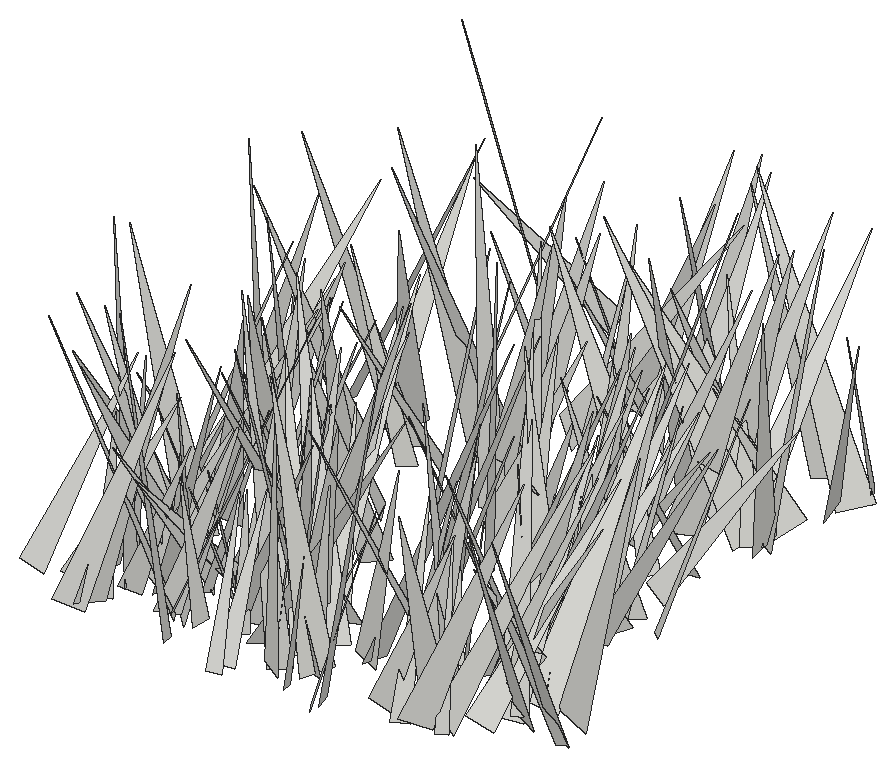
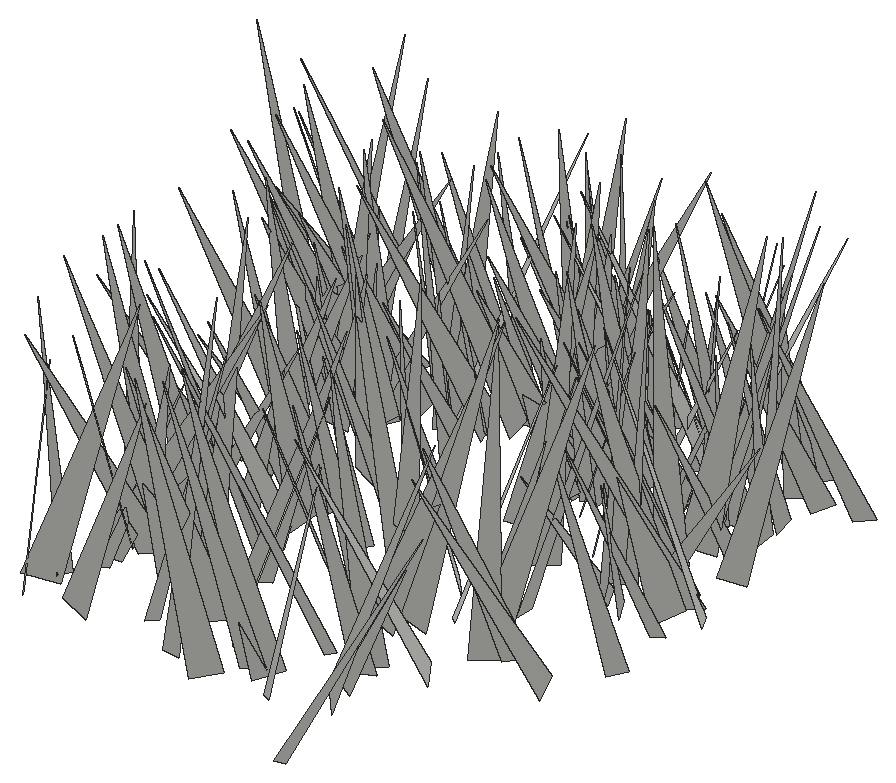
# SketchUp Ruby script. Lengths in inches.
U = 1.inch
M = Sketchup.active_model
def pt(a) = Geom::Point3d.new(a.map { |v| v * U })
def face(e, loops, mat)
  f = e.add_face(loops[0].map { |a| pt(a) })
  loops[1..].each { |l| e.add_face(l.map { |a| pt(a) }).erase! }
  f.material = f.back_material = mat if mat
  f
end
# faces: each face lists its corners as indices into pts; further lists are holes
def faces(e, pts, list, mat = nil) = list.each { |f| face(e, (f[0].is_a?(Array) ? f : [f]).map { |l| l.map { |i| pts[i] } }, mat) }
# xy, xz, yz: faces in a plane at the given z, y or x. An outline is a flat list of corners, or four numbers for a rectangle; further outlines are holes
def ring(l) = l.size == 4 ? [[l[0], l[1]], [l[2], l[1]], [l[2], l[3]], [l[0], l[3]]] : l.each_slice(2).to_a
def flat(e, list, mat, &to3) = list.each { |f| face(e, (f[0].is_a?(Array) ? f : [f]).map { |l| ring(l).map { |u, v| to3.(u, v) } }, mat) }
def xy(e, z, list, mat = nil) = flat(e, list, mat) { |x, y| [x, y, z] }
def xz(e, y, list, mat = nil) = flat(e, list, mat) { |x, z| [x, y, z] }
def yz(e, x, list, mat = nil) = flat(e, list, mat) { |y, z| [x, y, z] }
def lines(e, pts, list) = list.each { |a, b| e.add_line(pt(pts[a]), pt(pts[b])) }
# prism: a flat outline (further loops are holes) pulled along v
def prism(e, loops, v, mat = nil)
  f = face(e, loops, mat); d = Geom::Vector3d.new(v.map { |x| x * U })
  f.pushpull(f.normal.samedirection?(d) ? d.length : -d.length)
end
def box(e, o, s, mat = nil) = prism(e, [[o, [o[0] + s[0], o[1], o[2]], [o[0] + s[0], o[1] + s[1], o[2]], [o[0], o[1] + s[1], o[2]]]], [0, 0, s[2]], mat)
def at(x, y, z, deg = 0) = Geom::Transformation.translation(pt([x, y, z])) * Geom::Transformation.rotation(ORIGIN, Z_AXIS, deg.degrees)
def axes(o, x, y, z) = Geom::Transformation.new([*x, 0, *y, 0, *z, 0, *pt(o).to_a, 1])
def part(name) = M.definitions.add(name)
# library, detail: a bought-in or finely detailed component or shape, given as its bounding box
def library(name, o, s) = part(name).tap { |d| box(d.entities, o, s) }
def detail(e, o, s) = box(e.add_group.entities, o, s)
def put(e, d, t, mat = nil) = e.add_instance(d, t).tap { |i| i.material = mat if mat }
def group(e, t, mat = nil) = e.add_group.tap { |g| g.transformation = t; g.material = mat if mat }.entities
root = M.entities
c1 = part("fur_instance\#9")
p = [[0.8125,0,1.79],[0.67,-0.02,1.48],[0,-0.11,0],[0,0.11,0]]
faces(c1.entities,p,[[0,1,2,3]])
put(root,c1,axes([535.58,138.43,-21.86],[-0.09668,3.9627,0.07364],[3.92699,0.08582,0.53775],[-0.5359,-0.08606,3.92724]))
put(root,c1,axes([527.36,138.86,-21.66],[-2.26569,5.88907,2.62757],[5.5866,3.18358,-2.31806],[3.22106,-1.37923,5.86866]))
put(root,c1,axes([544.95,141.88,-21.86],[4.44508,-4.04211,0.97735],[-3.87336,-4.54492,-1.18043],[-1.51359,-0.24009,5.89101]))
put(root,c1,axes([537.28,140.2,-21.86],[-2.81459,-5.30869,2.75415],[-5.79641,3.17103,0.18862],[1.47279,2.33491,6.00571]))
put(root,c1,axes([550.42,143.29,-21.86],[-2.24137,-6.8028,0.2078],[-6.58087,2.22202,1.76064],[1.73594,-0.35988,6.94277]))
put(root,c1,axes([540.71,138.57,-21.86],[3.62249,2.81644,0.55831],[2.6251,-3.61284,1.19278],[-1.16313,0.61769,4.43081]))
put(root,c1,axes([535.55,139.2,-21.86],[-1.89071,3.52857,0.74513],[3.44423,2.01617,-0.80816],[1.06925,-0.25501,3.92077]))
put(root,c1,axes([539,141.21,-21.86],[-6.28621,2.90163,2.83322],[3.4688,6.55463,0.9835],[2.10096,-2.14018,6.85337]))
put(root,c1,axes([527.73,140.58,-21.86],[2.1664,-3.98299,1.68795],[-4.30586,-2.16689,0.41322],[-0.41582,1.68731,4.51516]))
put(root,c1,axes([531.38,141.05,-21.66],[-5.94217,-4.1756,0.21971],[-4.13273,5.80684,-1.41225],[-0.63601,1.27993,7.12394]))
put(root,c1,axes([542.83,140.66,-21.86],[1.73127,-4.9492,1.56465],[-4.93445,-1.0575,2.11492],[1.61056,2.08017,4.79781]))
put(root,c1,axes([545.28,140.01,-21.66],[4.70932,-5.02611,1.74089],[-5.27526,-4.11549,2.38842],[0.68127,2.87596,6.46026]))
put(root,c1,axes([532.46,139.17,-21.66],[-6.42625,-2.81034,1.42452],[-3.14557,5.90814,-2.53441],[0.18076,2.90169,6.53999]))
put(root,c1,axes([532.48,141.44,-21.86],[3.55115,-1.15094,1.45453],[-0.93925,-3.82501,-0.73353],[-1.59941,-0.30919,3.66022]))
put(root,c1,axes([548.5,143.38,-21.86],[-1.98153,-6.18192,0.39554],[-6.00617,2.01899,1.46585],[1.5161,-0.08133,6.32408]))
put(root,c1,axes([540.76,139.39,-21.86],[6.05789,3.57549,2.196],[3.19122,-6.43003,1.66595],[-2.72445,0.41853,6.83424]))
put(root,c1,axes([536.84,140.9,-21.86],[5.13574,3.88277,2.0176],[4.11622,-5.34233,-0.19668],[-1.48436,-1.3806,6.4353]))
put(root,c1,axes([527.87,139.65,-21.66],[7.54644,-1.30772,2.23251],[-1.88035,-7.50036,1.96263],[-1.77721,2.38276,7.40318]))
put(root,c1,axes([539.17,140.94,-21.86],[-4.91979,-5.33902,1.78444],[-5.59743,4.38767,-2.30455],[-0.5985,2.85253,6.88466]))
put(root,c1,axes([528.71,145.21,-21.86],[-6.90134,-2.30385,2.57209],[-0.73953,6.60101,3.92832],[3.37291,-3.26662,6.12409]))
put(root,c1,axes([530.66,144.61,-21.86],[-4.47086,-3.62986,0.22446],[-3.11938,4.01034,2.72058],[1.8697,-1.98902,5.07572]))
put(root,c1,axes([534,141.61,-21.86],[5.92157,-1.3609,0.111],[-1.36516,-5.91048,0.36315],[-0.02664,0.3788,6.06507]))
put(root,c1,axes([528.35,141.78,-21.86],[2.61538,-3.98544,0.72253],[-3.93735,-2.29982,1.56655],[0.95028,1.43982,4.50221]))
put(root,c1,axes([538.79,139.4,-21.86],[4.8815,3.3845,2.02519],[2.72156,-5.22275,2.16824],[-2.85471,0.80828,5.53015]))
put(root,c1,axes([531.01,141.01,-21.66],[4.31663,-3.25233,1.38409],[-3.53279,-4.03972,1.52536],[-0.11299,2.05661,5.185]))
put(root,c1,axes([534.42,141.6875,-21.86],[-2.65217,1.9255,1.58872],[2.09556,2.97695,-0.10973],[1.35655,-0.83418,3.2756]))
put(root,c1,axes([538.04,142.21,-21.86],[0.28341,4.29415,2.46111],[4.89058,0.13603,-0.80051],[0.76092,-2.47364,4.22839]))
put(root,c1,axes([525.99,140.88,-21.66],[3.23121,-4.00646,1.7311],[-4.24322,-2.37965,2.41277],[1.02152,2.78831,4.54653]))
put(root,c1,axes([546.67,140.04,-21.66],[0.48963,4.22721,0.04806],[3.94805,-0.47454,1.51627],[-1.51146,0.12987,3.97618]))
put(root,c1,axes([543.15,144.57,-21.86],[-5.31992,-4.92486,0.01845],[-4.88394,5.27914,0.91325],[0.63384,-0.65774,7.19179]))
put(root,c1,axes([524,140.59,-21.66],[-0.28996,5.60424,1.15409],[5.32871,0.68543,-1.98963],[2.08431,-0.97272,5.24719]))
put(root,c1,axes([531.73,141.1,-21.86],[3.18185,3.17768,0.5905],[3.1987,-3.21478,0.06397],[-0.46337,-0.37158,4.49642]))
put(root,c1,axes([540.14,143.03,-21.66],[-0.32261,-5.78503,1.74562],[-5.69921,0.87225,1.8374],[2.00818,1.5461,5.49497]))
put(root,c1,axes([536.28,144.05,-21.86],[2.99312,-6.69994,0.30324],[-6.59145,-2.87731,1.48788],[1.23852,0.87852,7.18569]))
put(root,c1,axes([544.47,140,-21.86],[-4.53148,2.02632,0.31118],[1.79338,4.28391,-1.78018],[0.99329,1.50971,4.63371]))
put(root,c1,axes([531.27,142.54,-21.86],[4.09073,2.15745,2.5023],[2.51133,-4.61824,-0.12369],[-2.14694,-1.2913,4.62314]))
put(root,c1,axes([531.03,145.58,-21.86],[-4.31312,-2.31019,0.44376],[-1.59331,3.55068,2.99849],[1.73068,-2.4885,3.8664]))
put(root,c1,axes([546.14,140.92,-21.66],[3.48936,7.09192,0.65775],[6.9322,-3.21357,-2.12629],[1.63479,-1.51038,7.61247]))
put(root,c1,axes([535.52,141.73,-21.86],[6.82569,-2.14516,0.01525],[-2.06759,-6.56497,1.95405],[0.57187,1.86856,6.88284]))
put(root,c1,axes([537.53,140.48,-21.86],[0.70112,8.01126,1.73468],[7.49163,-1.33281,3.12731],[-3.32639,-1.31314,7.4089]))
put(root,c1,axes([529.29,142.86,-21.86],[6.44978,-0.00096,0.92482],[0.04605,-6.50733,-0.32793],[-0.92367,-0.33115,6.44144]))
put(root,c1,axes([536.25,143.45,-21.86],[6.7511,0.38921,2.10678],[0.68602,-6.99103,-0.90679],[-2.02963,-1.06837,6.70124]))
put(root,c1,axes([532.49,143.96,-21.86],[-2.2334,-3.12116,0.78897],[-3.02774,2.36275,0.77617],[1.09405,0.16724,3.75863]))
put(root,c1,axes([537.57,145.16,-21.66],[-1.57704,-7.74459,0.50786],[-7.45096,1.36569,-2.31124],[-2.17253,0.93802,7.55804]))
put(root,c1,axes([533.32,143.04,-21.86],[-3.78552,-3.06993,0.30173],[-3.01727,3.58565,-1.37288],[-0.64154,1.25071,4.67652]))
put(root,c1,axes([550.98,142.79,-21.86],[-3.53185,-5.19128,1.06072],[-4.89285,2.7062,-3.04713],[-2.03336,2.50511,5.48984]))
put(root,c1,axes([545.41,142.875,-21.86],[3.76786,2.01641,1.4087],[2.07515,-3.9894,0.15999],[-1.32064,-0.51569,4.27049]))
put(root,c1,axes([528.1,143.29,-21.86],[1.52671,4.77623,1.67607],[4.63081,-0.61106,-2.47682],[2.04382,-2.18327,4.35989]))
put(root,c1,axes([533.61,143.32,-21.86],[-0.36242,4.3186,2.109],[4.6668,0.82166,-0.88056],[1.14855,-1.97588,4.24338]))
put(root,c1,axes([537.66,142.11,-21.86],[-3.34888,5.66427,0.75226],[5.70524,3.26636,0.80369],[-0.31635,-1.05439,6.53093]))
put(root,c1,axes([528.13,145.96,-21.86],[-7.13222,-2.21187,1.52983],[-1.72076,7.08542,2.22194],[2.06682,-1.73369,7.12909]))
put(root,c1,axes([530.79,141.89,-21.86],[7.17048,3.0592,0.30714],[3.02615,-7.16002,0.66735],[-0.54355,0.49421,7.76718]))
put(root,c1,axes([528.59,144.34,-21.86],[-1.07299,-3.39329,1.1863],[-3.30809,1.41653,1.05972],[1.4065,0.74301,3.39746]))
put(root,c1,axes([528.04,142.3,-21.86],[-7.59721,-1.99805,2.32928],[-2.54922,7.5713,-1.81993],[1.70857,2.41215,7.64184]))
put(root,c1,axes([528.81,144.4,-21.66],[1.01091,-5.94061,2.30759],[-6.04054,-1.63799,-1.57056],[-2.03168,1.91413,5.81775]))
put(root,c1,axes([526.56,142.86,-21.86],[5.06172,0.87175,1.3003],[0.68802,-5.19178,0.80241],[-1.40619,0.59773,5.07318]))
put(root,c1,axes([546.61,143.11,-21.66],[3.72746,5.46093,0.78491],[5.42353,-3.45332,-1.72965],[1.01153,-1.60767,6.38153]))
put(root,c1,axes([534.61,140.5,-21.66],[5.37795,5.75,0.47067],[5.40496,-5.24661,2.33794],[-2.01755,1.27162,7.51791]))
put(root,c1,axes([542.57,144.18,-21.86],[-2.5167,4.57974,3.46384],[4.9953,3.61127,-1.14527],[2.83182,-2.30014,5.09864]))
put(root,c1,axes([550.05,144.65,-21.86],[2.12208,6.92928,3.4126],[7.54208,-1.09525,-2.46604],[1.66665,-3.86645,6.81445]))
put(root,c1,axes([536.61,144.58,-21.86],[4.26627,1.55205,0.05399],[1.49304,-4.05567,-1.39111],[0.42732,-1.32496,4.32143]))
put(root,c1,axes([535.61,142.67,-21.86],[-0.37252,4.33667,0.3989],[4.3129,0.31185,0.63743],[-0.60398,-0.44793,4.30572]))
put(root,c1,axes([548.32,146.01,-21.66],[2.70067,-3.13661,0.88183],[-2.51329,-2.73437,-2.02883],[-2.07348,-0.77102,3.60774]))
put(root,c1,axes([545.52,145.23,-21.86],[5.8756,3.65861,0.2575],[3.32747,-5.11292,-3.2803],[1.54262,-2.90637,6.0949]))
put(root,c1,axes([541.43,144.65,-21.66],[3.4231,3.63538,1.50249],[3.93251,-3.11512,-1.42212],[0.09387,-2.06666,4.78656]))
put(root,c1,axes([543.79,144.3,-21.86],[-6.14594,-1.15799,1.95321],[-1.28361,6.42082,-0.2323],[1.87305,0.60056,6.24977]))
put(root,c1,axes([526.43,144.3,-21.86],[4.53301,0.32886,1.81446],[0.26511,-4.88148,0.22244],[-1.82486,0.10775,4.53948]))
put(root,c1,axes([525.06,148.28,-21.66],[5.40671,-4.03304,0.21931],[-3.53675,-4.90438,-2.9974],[-1.95061,-2.2864,6.04264]))
put(root,c1,axes([537.93,143.39,-21.86],[-3.99948,7.12267,1.32626],[7.23474,3.8453,1.16596],[-0.38726,-1.72292,8.0851]))
put(root,c1,axes([536.92,145.22,-21.86],[-3.87014,-4.65436,0.40491],[-4.4497,3.51193,-2.16136],[-1.42379,1.67578,5.65416]))
put(root,c1,axes([547.15,142.01,-21.86],[-2.23637,5.81255,0.47787],[5.16217,2.21098,-2.73477],[2.71405,0.58421,5.59536]))
put(root,c1,axes([540.44,143.29,-21.66],[8.13769,0.92636,1.08085],[0.65484,-8.00564,1.93114],[-1.26395,1.81658,7.95932]))
put(root,c1,axes([531,143.68,-21.86],[3.99187,0.97882,1.10255],[0.50795,-3.90054,1.62373],[-1.38409,1.39155,3.77579]))
put(root,c1,axes([547.1,143.93,-21.86],[0.14678,4.73777,0.12743],[4.7339,-0.15274,0.22615],[-0.23006,-0.12022,4.73465]))
put(root,c1,axes([534.15,142.83,-21.86],[6.07778,0.82962,2.17123],[-0.33597,-5.70106,3.1188],[-2.29992,3.02515,5.28212]))
put(root,c1,axes([543.09,145.43,-21.86],[-1.02276,3.4571,1.0392],[3.60758,1.01767,0.16502],[0.12981,-1.04418,3.60144]))
put(root,c1,axes([546.28,146.38,-21.86],[-4.22462,-4.77942,0.40733],[-4.62488,3.91455,-2.0354],[-1.27248,1.63999,6.04544]))
put(root,c1,axes([546.88,145.61,-21.86],[-3.59286,-3.26733,2.03566],[-3.70516,3.69058,-0.61592],[1.04455,1.85261,4.81713]))
put(root,c1,axes([527.9,147.04,-21.66],[2.50523,-6.92108,2.84903],[-7.08461,-3.16179,-1.45116],[-2.41383,2.09672,7.21607]))
put(root,c1,axes([548.07,143.15,-21.66],[0.30584,8.28043,0.48557],[7.987,-0.4251,2.21855],[-2.2381,-0.38549,7.98355]))
put(root,c1,axes([541.33,147.29,-21.66],[6.22131,1.299,1.34326],[1.60809,-6.10017,-1.54868],[-0.95174,-1.81575,6.1639]))
put(root,c1,axes([545.39,146.73,-21.86],[6.11915,-4.70581,1.11272],[-4.83462,-5.98952,1.25659],[-0.09634,1.67568,7.61641]))
put(root,c1,axes([547.87,143.1,-21.86],[-4.8564,4.18897,0.42907],[3.70643,4.56321,-2.59917],[1.99849,1.71635,5.86314]))
put(root,c1,axes([532.84,144.54,-21.66],[-6.71814,2.72987,2.53139],[2.23652,7.13443,-1.75826],[2.97626,0.8008,7.03521]))
put(root,c1,axes([527.91,148.82,-21.66],[2.36593,-6.95857,0.28973],[-6.83072,-2.25873,1.53056],[1.359,0.76137,7.18865]))
put(root,c1,axes([548.5625,145.07,-21.66],[-4.5247,0.14497,1.56827],[-0.47946,4.4174,-1.79167],[1.5002,1.84904,4.15738]))
put(root,c1,axes([534.73,145.96,-21.66],[7.47756,-1.51643,1.55812],[-1.8154,-7.42558,1.48539],[-1.19651,1.78955,7.48379]))
put(root,c1,axes([534.18,146.23,-21.86],[-1.06035,5.5551,1.84187],[5.77115,1.30347,-0.60889],[0.97234,-1.67863,5.62252]))
put(root,c1,axes([536.57,145.66,-21.86],[-2.34195,3.99616,0.3444],[3.99913,2.35703,-0.15486],[0.30802,-0.21845,4.62925]))
put(root,c1,axes([544.57,145.09,-21.86],[8.0865,0.10169,1.15451],[-0.2162,-7.86244,2.20681],[-1.13864,2.21504,7.78021]))
put(root,c1,axes([526.5625,146.26,-21.86],[4.0884,0.15219,0.34801],[0.0557,-3.96154,1.07814],[-0.37573,1.0688,3.94662]))
put(root,c1,axes([534.61,145.07,-21.66],[-3.66435,5.27166,1.90181],[4.6134,4.12758,-2.55233],[3.18179,0.08644,5.89097]))
put(root,c1,axes([541.47,144.17,-21.66],[7.3603,1.92647,1.4977],[1.22652,-7.03518,3.02165],[-2.10951,2.63124,6.98247]))
put(root,c1,axes([547.6,146.57,-21.86],[-6.9298,2.98954,1.57704],[3.02348,7.09089,-0.15622],[1.51094,-0.47802,7.54553]))
put(root,c1,axes([548.91,146.2,-21.86],[-2.11834,3.44874,0.2067],[3.45458,2.11778,0.0692],[0.04913,-0.21236,4.04678]))
put(root,c1,axes([533.68,145.81,-21.66],[-6.0255,1.4926,2.28597],[0.94971,6.33899,-1.63567],[2.5596,1.16168,5.98825]))
put(root,c1,axes([530.72,146.12,-21.86],[4.2696,-0.12633,0.87704],[-0.45536,-4.01534,1.6384],[-0.76014,1.6958,3.94476]))
put(root,c1,axes([546.43,145.24,-21.86],[7.47336,0.82298,1.26079],[0.38429,-7.21504,2.43175],[-1.45575,2.3203,7.11442]))
put(root,c1,axes([548.43,144.48,-21.66],[-1.16046,8.00046,0.20395],[7.87345,1.17823,-1.41992],[1.43448,0.00519,7.95851]))
put(root,c1,axes([535.15,150.01,-21.66],[2.99002,-5.93259,1.12286],[-5.76165,-3.17812,-1.449],[-1.8055,0.31717,6.48354]))
put(root,c1,axes([531.17,150.04,-21.66],[-4.0085,-3.44331,0.94309],[-3.06456,4.04605,1.74695],[1.83147,-0.76613,4.98725]))
put(root,c1,axes([534.1,147,-21.66],[-5.43034,-1.89464,0.64767],[-1.9986,5.01546,-2.08529],[-0.12137,2.18018,5.36002]))
put(root,c1,axes([541.21,146.23,-21.66],[4.47299,1.54799,0.88013],[1.09405,-4.26651,1.94385],[-1.40498,1.60599,4.31572]))
put(root,c1,axes([528.74,151.34,-21.66],[6.44625,-4.17663,0.34492],[-3.99481,-6.31514,-1.81045],[-1.26676,-1.33867,7.46462]))
put(root,c1,axes([527.57,149.45,-21.66],[-0.38653,-3.78857,0.47263],[-3.40937,0.1287,-1.7566],[-1.71837,0.59684,3.37891]))
put(root,c1,axes([545.21,146.82,-21.66],[-6.19625,3.45387,1.64148],[3.0912,6.3638,-1.72156],[2.25127,0.76815,6.88178]))
put(root,c1,axes([535.02,147.12,-21.66],[5.43487,-1.88004,3.06705],[-2.9758,-5.47185,1.91904],[-2.02138,3.00059,5.42123]))
put(root,c1,axes([546.625,148.18,-21.66],[-1.63602,4.97918,0.62205],[4.87533,1.42244,1.43652],[-1.18757,-1.0199,5.04036]))
put(root,c1,axes([547.03,151.7,-21.66],[2.87484,-4.36178,0.57915],[-3.91954,-2.85297,-2.03053],[-1.99945,-0.67874,4.81319]))
put(root,c1,axes([535.59,145.8125,-21.66],[-4.59589,5.78444,0.11594],[5.4804,4.40003,-2.28044],[1.8543,1.33244,7.02721]))
put(root,c1,axes([532.2,152.1,-21.66],[6.58115,-3.41587,1.26301],[-3.10443,-6.62563,-1.74311],[-1.90417,-1.00387,7.20703]))
put(root,c1,axes([547.16,146.14,-21.86],[-6.41092,4.00729,0.82453],[3.32918,6.00061,-3.27831],[2.37798,2.40258,6.81256]))
put(root,c1,axes([543.35,149.74,-21.66],[2.52048,5.79703,1.2985],[5.75928,-2.03853,-2.07834],[1.45681,-1.97061,5.96983]))
put(root,c1,axes([525.625,149.92,-21.66],[4.10268,4.53992,0.30052],[4.35228,-3.79801,-2.04106],[1.3262,-1.58032,5.76861]))
put(root,c1,axes([546.86,150.13,-21.66],[5.8068,-2.41673,0.19711],[-2.36119,-5.5195,1.88633],[0.55156,1.81463,6.0001]))
put(root,c1,axes([525.98,150.53,-21.66],[3.52755,5.08967,0.59914],[4.90233,-3.13928,-2.19532],[1.49362,-1.71683,5.79042]))
put(root,c1,axes([543.72,152.17,-21.66],[4.89387,1.35478,0.49174],[1.44124,-4.60961,-1.64362],[-0.00784,-1.71558,4.80457]))
put(root,c1,axes([528.08,153.29,-21.66],[-6.05203,-3.65216,2.90127],[-3.20675,6.70926,1.75646],[3.38709,-0.1736,6.84691]))
put(root,c1,axes([532.67,153.53,-21.66],[-3.8372,-2.33717,0.79383],[-2.01321,3.81242,1.493],[1.42812,-0.90538,4.23762]))
put(root,c1,axes([523.78,151.76,-21.66],[5.98281,3.47845,0.55141],[3.51313,-5.81778,-1.41742],[0.2481,-1.50052,6.77381]))
put(root,c1,axes([545.11,152.66,-21.66],[0.56131,-6.10589,2.64479],[-6.41112,0.21442,1.85565],[1.78167,2.69518,5.8441]))
put(root,c1,axes([527.89,151.6,-21.66],[3.6249,6.4726,3.15784],[6.5149,-4.45394,1.65071],[-3.06961,-1.8095,7.23254]))
put(root,c1,axes([546.875,152.97,-21.66],[-1.11932,5.12608,2.18052],[5.30702,0.30525,2.00664],[-1.6932,-2.43194,4.84799]))
put(root,c1,axes([525.21,152.33,-21.66],[6.77248,-2.83159,1.61361],[-3.13932,-6.6674,1.47599],[-0.87537,2.00399,7.19067]))
put(root,c1,axes([530.27,155.84,-21.66],[-7.65526,-2.65251,1.50577],[-2.23878,7.64939,2.09305],[2.07148,-1.53532,7.82675]))
put(root,c1,axes([524.98,151.12,-21.66],[0.81957,8.13408,0.73803],[7.68253,-0.51597,-2.84467],[2.77248,-0.97476,7.66439]))
put(root,c1,axes([542.63,154.875,-21.66],[2.44609,-6.94499,1.47158],[-6.99231,-2.08787,1.76924],[1.22722,1.94671,7.14745]))
put(root,c1,axes([542.59,151,-21.66],[1.27817,7.72916,0.81529],[7.27012,-1.48113,2.64386],[-2.74773,-0.32349,7.37453]))
put(root,c1,axes([539.55,152.16,-21.66],[-6.21182,-1.68937,2.27799],[-2.42044,6.01654,-2.13837],[1.47806,2.75267,6.07191]))
put(root,c1,axes([537.28,152.08,-21.66],[5.41894,2.39891,1.8987],[1.67708,-5.5593,2.23748],[-2.55876,1.4367,5.48756]))
put(root,c1,axes([528.24,152.49,-21.66],[3.83996,1.68055,0.1423],[1.49178,-3.54944,1.66307],[-0.78682,1.47206,3.84756]))
put(root,c1,axes([546.59,152.37,-21.66],[2.63197,4.07891,0.20518],[3.86496,-2.5665,1.44292],[-1.31973,0.61842,4.63495]))
put(root,c1,axes([527.16,153.14,-21.66],[3.31155,2.43431,1.59522],[1.82743,-3.61986,1.73033],[-2.2652,0.63849,3.72802]))
put(root,c1,axes([524.55,153.92,-21.66],[1.36791,4.73736,0.76135],[4.55305,-1.0318,-1.76027],[1.51392,-1.17738,4.60599]))
put(root,c1,axes([542.03,154.02,-21.66],[3.72107,-3.56028,1.90501],[-4.03778,-3.30047,1.71878],[-0.03061,2.5656,4.85467]))
put(root,c1,axes([539.13,155.61,-21.66],[1.54528,-3.8993,0.59524],[-3.77652,-1.27799,1.43226],[1.13873,1.05307,3.94222]))
put(root,c1,axes([548.45,152.37,-21.66],[3.88995,3.95886,0.07672],[3.75671,-3.72392,1.68217],[-1.25122,1.12695,5.2891]))
put(root,c1,axes([537.33,154.94,-21.66],[1.43912,5.66343,2.07225],[5.60003,-0.46439,-2.61988],[2.23794,-2.47985,5.22319]))
put(root,c1,axes([544.11,152.97,-21.66],[-0.54715,4.89077,0.10405],[4.53126,0.54616,-1.84371],[1.84341,0.10915,4.56287]))
put(root,c1,axes([532.22,158.19,-21.66],[-4.33714,-4.09832,0.0827],[-3.81397,4.0787,2.10515],[1.50223,-1.4771,5.58349]))
put(root,c1,axes([535.85,157.02,-21.66],[-0.11111,-7.60969,2.49454],[-7.52897,0.94928,2.56048],[2.72852,2.30953,7.16685]))
put(root,c1,axes([546.19,155.13,-21.66],[1.31269,5.55847,0.82299],[4.82858,-0.68361,-3.08457],[2.8738,-1.39037,4.80678]))
put(root,c1,axes([543.68,154.3,-21.66],[-1.09311,5.26549,0.63584],[5.05113,1.23151,-1.51458],[1.61731,-0.28736,5.16007]))
put(root,c1,axes([546.5,157.39,-21.66],[-1.81586,-4.37557,0.34615],[-4.20637,1.62778,-1.48984],[-1.25376,0.87607,4.49704]))
put(root,c1,axes([544.98,156.3,-21.66],[-1.55107,4.41542,0.77186],[4.34501,1.28043,1.40671],[-1.10114,-1.16708,4.46351]))
put(root,c1,axes([523.87,157.54,-21.66],[2.085,-4.49657,0.98747],[-4.39792,-1.62495,1.88661],[1.36107,1.63764,4.58334]))
put(root,c1,axes([530.97,157.29,-21.66],[-1.13244,4.66111,1.93868],[4.91983,0.57378,1.4943],[-1.13125,-2.17064,4.55801]))
put(root,c1,axes([529.06,160.03,-21.66],[6.38115,-3.67921,0.2036],[-3.55943,-6.25987,-1.56256],[-0.95316,-1.25481,7.1982]))
put(root,c1,axes([536.32,156.49,-21.66],[0.66704,7.88186,2.68055],[8.14998,-1.16705,1.40349],[-1.69907,-2.50365,7.78452]))
put(root,c1,axes([529.87,158.65,-21.66],[-0.48012,-7.554,2.16495],[-7.6037,-0.10085,-2.03814],[-1.98335,2.21526,7.28968]))
put(root,c1,axes([533.84,155.71,-21.66],[3.8094,4.08661,1.06154],[3.80016,-3.94157,1.53675],[-1.84012,0.32005,5.37125]))
put(root,c1,axes([542.66,157.85,-21.66],[2.65844,-2.5721,0.0216],[-2.2994,-2.3625,1.67773],[1.15278,1.21916,3.2967]))
put(root,c1,axes([542.42,155.59,-21.66],[-6.84761,2.51212,1.52779],[1.98246,6.80446,-2.30302],[2.17135,1.70976,6.92074]))
put(root,c1,axes([534.45,160.42,-21.66],[-1.86183,-7.54983,1.10161],[-7.50699,1.61006,-1.65309],[-1.3633,1.44488,7.59827]))
put(root,c1,axes([533.54,159.5,-21.66],[-0.98581,-7.65367,2.64082],[-7.9173,0.35473,-1.92744],[-1.69382,2.79641,7.47232]))
put(root,c1,axes([547.21,161.26,-21.66],[7.02659,-0.33713,1.59],[0.09653,-6.95626,-1.90152],[-1.62247,-1.87389,6.7728]))
put(root,c1,axes([542.24,158.82,-21.66],[3.65176,6.04586,1.11201],[6.02251,-3.25936,-2.05677],[1.23222,-1.98709,6.75703]))
put(root,c1,axes([542.32,156.81,-21.66],[7.12213,3.78972,1.00867],[3.4176,-7.02352,2.25704],[-1.92338,1.55314,7.74548]))
put(root,c1,axes([546.34,161.41,-21.66],[-7.92246,2.32052,1.49756],[2.68865,7.5204,2.57051],[0.63138,-2.90715,7.84491]))
put(root,c1,axes([542.16,162.46,-21.66],[-1.3783,-7.92591,0.91068],[-7.76861,1.54372,1.6777],[1.81604,0.58822,7.86798]))
put(root,c1,axes([540.83,160.8125,-21.66],[-5.87282,3.13064,1.60123],[3.47052,5.66214,1.65846],[0.56601,-2.23474,6.44519]))
put(root,c1,axes([534.95,160.33,-21.66],[-0.35143,6.05342,2.99786],[6.31844,1.35633,-1.99808],[2.38924,-2.69649,5.72495]))
put(root,c1,axes([543.76,159.93,-21.66],[6.10397,-4.61293,1.81963],[-4.95361,-5.80478,1.9013],[-0.22786,2.62185,7.41098]))
put(root,c1,axes([538.9,158.21,-21.66],[2.7978,5.22834,0.27095],[4.99402,-2.75746,1.64099],[-1.57121,0.54549,5.69828]))
put(root,c1,axes([547.18,163.09,-21.66],[-6.27712,3.42033,1.55819],[3.73626,5.34865,3.31076],[-0.40863,-3.63622,6.33559]))
put(root,c1,axes([527.99,159.18,-21.66],[-2.51338,5.74575,1.01303],[5.46798,2.70448,-1.77311],[2.03497,-0.17044,6.01555]))
put(root,c1,axes([546.6875,163.89,-21.66],[-4.22388,-0.55824,1.0602],[-0.01996,3.91714,1.98304],[1.19803,-1.90295,3.77099]))
put(root,c1,axes([543.84,162.39,-21.66],[4.37755,-6.1842,1.75356],[-6.40379,-4.01166,1.83857],[0.55746,2.47882,7.3503]))
put(root,c1,axes([546.74,160.91,-21.66],[-0.83276,5.81039,0.96307],[5.68734,0.54058,1.65638],[-1.53047,-1.15272,5.63121]))
put(root,c1,axes([532.32,163.48,-21.66],[1.87666,-6.19619,1.68038],[-6.32701,-1.4881,1.57887],[1.08876,2.03251,6.27868]))
put(root,c1,axes([525.49,160.35,-21.66],[6.20269,2.14266,0.41588],[1.88774,-5.89525,2.21806],[-1.09562,1.97291,6.17613]))
put(root,c1,axes([538.27,165.57,-21.66],[-4.62318,-3.47557,0.41553],[-3.19467,4.47097,1.85217],[1.4305,-1.24775,5.47931]))
put(root,c1,axes([544.24,161.7,-21.66],[-0.17327,7.80384,1.95788],[7.72096,0.71202,-2.15474],[2.26272,-1.83203,7.50246]))
put(root,c1,axes([547.47,161.14,-21.66],[3.93388,5.26717,1.14139],[4.90502,-4.08461,1.94372],[-2.23307,0.30691,6.28017]))
put(root,c1,axes([542.2,166.18,-21.66],[-5.45284,-1.57742,1.94379],[-0.6971,5.43147,2.45217],[2.40429,-2.00271,5.11943]))
put(root,c1,axes([547.57,165.37,-21.66],[5.98567,0.36805,0.66862],[0.55714,-5.71998,-1.83907],[-0.52163,-1.88604,5.70802]))
put(root,c1,axes([534.47,163.69,-21.66],[4.68753,6.76488,0.69054],[6.04009,-3.75687,-4.19721],[3.12373,-2.88717,7.07954]))
put(root,c1,axes([532.27,164.22,-21.66],[0.67083,5.9533,2.27987],[6.17356,-0.03505,-1.72498],[1.58958,-2.37626,5.73727]))
put(root,c1,axes([545.71,161.52,-21.66],[-2.00066,7.03095,0.19663],[6.73059,1.97306,-2.06922],[2.04255,0.38513,7.01108]))
put(root,c1,axes([539.76,167.95,-21.66],[-3.16207,-7.07316,1.24758],[-6.76016,3.39142,2.09364],[2.42619,0.2311,7.45956]))
put(root,c1,axes([530.11,162.48,-21.66],[5.9455,4.2001,0.21568],[4.05072,-5.81939,1.66213],[-1.13095,1.23699,7.08711]))
put(root,c1,axes([532.14,165.71,-21.66],[-1.49858,-3.44059,1.04989],[-3.40031,0.98374,-1.62968],[-1.17382,1.54281,3.38047]))
put(root,c1,axes([548,167.68,-21.66],[-3.52584,-3.38703,1.52089],[-2.9555,3.82986,1.67745],[2.24724,-0.27722,4.59235]))
put(root,c1,axes([548.17,166.3,-21.66],[-5.06971,5.94983,1.91077],[6.22333,4.58369,2.23904],[-0.56711,-2.88838,7.48926]))
put(root,c1,axes([535.36,166.82,-21.66],[5.33015,-4.46349,0.382],[-4.4244,-5.15196,1.5366],[0.7024,1.41905,6.78027]))
put(root,c1,axes([534.23,168.37,-21.66],[-3.15103,-4.03715,0.66571],[-3.75697,3.18756,1.54769],[1.62077,-0.46003,4.88182]))
put(root,c1,axes([540,164.43,-21.66],[-2.57926,6.41675,1.59968],[6.21683,2.93816,-1.76197],[2.25493,-0.76079,6.68751]))
put(root,c1,axes([532.0625,166.77,-21.66],[-6.33694,-5.31771,1.42218],[-5.44687,5.74429,-2.79146],[-0.79519,3.03026,7.78734]))
put(root,c1,axes([536.2,166.79,-21.66],[0.74046,6.81709,2.01452],[6.9144,-0.22063,-1.79488],[1.64984,-2.13492,6.61811]))
put(root,c1,axes([545.39,167.48,-21.66],[-0.37721,6.24874,2.25952],[6.16262,-0.51732,2.45945],[-2.4848,-2.23161,5.75674]))
put(root,c1,axes([537.4,168.49,-21.66],[3.87683,-5.48097,2.21285],[-5.90731,-3.50163,1.67625],[0.20355,2.76859,6.50085]))
put(root,c1,axes([530.3,172.39,-21.66],[-5.57045,-1.42182,0.3414],[-1.0257,4.7578,3.07884],[1.04215,-2.91715,4.85512]))
